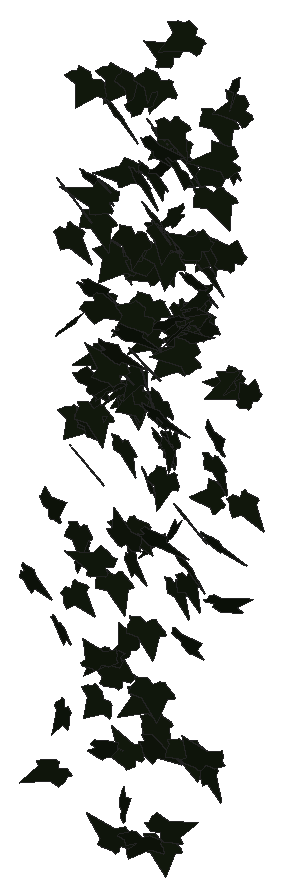
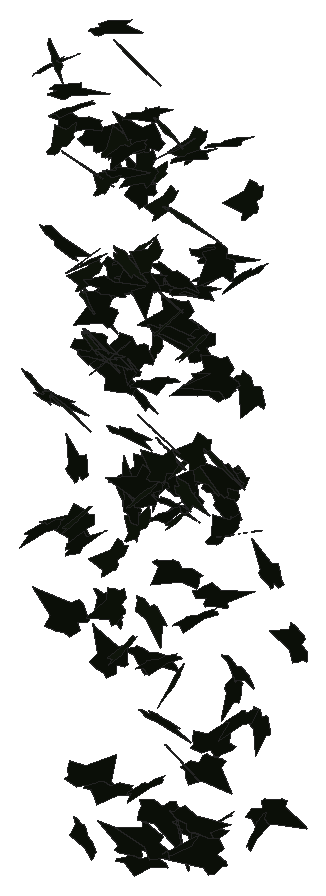
# SketchUp Ruby script. Lengths in inches.
U = 1.inch
M = Sketchup.active_model
def pt(a) = Geom::Point3d.new(a.map { |v| v * U })
def face(e, loops, mat)
  f = e.add_face(loops[0].map { |a| pt(a) })
  loops[1..].each { |l| e.add_face(l.map { |a| pt(a) }).erase! }
  f.material = f.back_material = mat if mat
  f
end
# faces: each face lists its corners as indices into pts; further lists are holes
def faces(e, pts, list, mat = nil) = list.each { |f| face(e, (f[0].is_a?(Array) ? f : [f]).map { |l| l.map { |i| pts[i] } }, mat) }
# xy, xz, yz: faces in a plane at the given z, y or x. An outline is a flat list of corners, or four numbers for a rectangle; further outlines are holes
def ring(l) = l.size == 4 ? [[l[0], l[1]], [l[2], l[1]], [l[2], l[3]], [l[0], l[3]]] : l.each_slice(2).to_a
def flat(e, list, mat, &to3) = list.each { |f| face(e, (f[0].is_a?(Array) ? f : [f]).map { |l| ring(l).map { |u, v| to3.(u, v) } }, mat) }
def xy(e, z, list, mat = nil) = flat(e, list, mat) { |x, y| [x, y, z] }
def xz(e, y, list, mat = nil) = flat(e, list, mat) { |x, z| [x, y, z] }
def yz(e, x, list, mat = nil) = flat(e, list, mat) { |y, z| [x, y, z] }
def lines(e, pts, list) = list.each { |a, b| e.add_line(pt(pts[a]), pt(pts[b])) }
# prism: a flat outline (further loops are holes) pulled along v
def prism(e, loops, v, mat = nil)
  f = face(e, loops, mat); d = Geom::Vector3d.new(v.map { |x| x * U })
  f.pushpull(f.normal.samedirection?(d) ? d.length : -d.length)
end
def box(e, o, s, mat = nil) = prism(e, [[o, [o[0] + s[0], o[1], o[2]], [o[0] + s[0], o[1] + s[1], o[2]], [o[0], o[1] + s[1], o[2]]]], [0, 0, s[2]], mat)
def at(x, y, z, deg = 0) = Geom::Transformation.translation(pt([x, y, z])) * Geom::Transformation.rotation(ORIGIN, Z_AXIS, deg.degrees)
def axes(o, x, y, z) = Geom::Transformation.new([*x, 0, *y, 0, *z, 0, *pt(o).to_a, 1])
def part(name) = M.definitions.add(name)
# library, detail: a bought-in or finely detailed component or shape, given as its bounding box
def library(name, o, s) = part(name).tap { |d| box(d.entities, o, s) }
def detail(e, o, s) = box(e.add_group.entities, o, s)
def put(e, d, t, mat = nil) = e.add_instance(d, t).tap { |i| i.material = mat if mat }
def group(e, t, mat = nil) = e.add_group.tap { |g| g.transformation = t; g.material = mat if mat }.entities
root = M.entities
M.materials.add("1026 AP 7946 SUNNY SIDE UP").color = [254, 231, 186]
M.materials.add("efeu1").color = [18, 25, 13]
c1 = part("ivyleaf_9")
p = [[1.54,2.16,1.25],[1.36,2.04,1.19],[-0.21,0.99,0.68],[-0.71,1.11,0.82],[-0.85,0.86,0.67],[-0.8,0.17,0.21],
  [-0.9,-0.01,0.1],[-0.67,-0.16,-0.02],[-0.08,-0.08,-0.05],[-0.03,-0.6,-0.4],[0.65,-0.88,-0.66],[0.83,-0.6,-0.49],
  [1.29,-0.42,-0.43],[1.8125,-0.07,-0.26],[1.21,0.44,0.15]]
faces(c1.entities,p,[[0,1,2,3,4,5,6,7,8,9,10,11,12,13,14]],"efeu1")
put(root,c1,axes([168.82,210.77,309.2],[-0.44916,-0.2938,0.16947],[0.00239,-0.21881,-0.39713],[0.53074,-0.24766,0.14521]),"1026 AP 7946 SUNNY SIDE UP")
put(root,c1,axes([168.69,210.7,304.06],[-0.41014,-0.05137,-0.32784],[0.50445,-0.00547,-0.27027],[0.04453,-0.41121,0.04211]),"1026 AP 7946 SUNNY SIDE UP")
put(root,c1,axes([168.9375,210.49,303.13],[0.06762,-0.09449,-0.44363],[-0.43394,0.33096,-0.10139],[0.53956,0.27802,-0.02595]),"1026 AP 7946 SUNNY SIDE UP")
put(root,c1,axes([168.94,211.13,324.72],[-0.38736,-0.37553,0.13039],[-0.00621,-0.14914,-0.45698],[0.62417,-0.23454,0.07638]),"1026 AP 7946 SUNNY SIDE UP")
put(root,c1,axes([169.12,209.28,314.23],[0.11699,0.37991,0.23372],[0.10984,0.21488,-0.39682],[-0.6853,0.0993,-0.0237]),"1026 AP 7946 SUNNY SIDE UP")
put(root,c1,axes([169.49,211.05,312.21],[-0.50728,0.27598,0.01138],[-0.05199,-0.02414,-0.43558],[-0.43108,-0.32185,0.03915]),"1026 AP 7946 SUNNY SIDE UP")
put(root,c1,axes([168.85,211.18,320.21],[0.70778,-0.08409,-0.10764],[-0.17067,-0.0163,-0.47045],[0.12289,0.4617,-0.03342]),"1026 AP 7946 SUNNY SIDE UP")
put(root,c1,axes([168.6,207.34,303.48],[0.19237,-0.05459,-0.43971],[0.67578,0.02942,0.12329],[0.02118,-0.44273,0.05977]),"1026 AP 7946 SUNNY SIDE UP")
put(root,c1,axes([168.95,209.93,301.71],[0.16673,-0.27771,-0.32909],[-0.12089,0.30956,-0.30322],[0.6526,0.12829,0.02791]),"1026 AP 7946 SUNNY SIDE UP")
put(root,c1,axes([169.16,210.78,309.1],[-0.26105,-0.17459,0.42549],[0.43389,0.30871,0.24991],[-0.55757,0.32197,-0.00473]),"1026 AP 7946 SUNNY SIDE UP")
put(root,c1,axes([169.3,208.57,300.82],[0.46262,-0.09432,-0.3028],[-0.46182,0.03704,-0.31547],[0.14676,0.41384,-0.03821]),"1026 AP 7946 SUNNY SIDE UP")
put(root,c1,axes([169.2,209.03,296.68],[0.06619,-0.08624,-0.47588],[0.47183,-0.35134,0.09379],[-0.56764,-0.30209,0.02247]),"1026 AP 7946 SUNNY SIDE UP")
put(root,c1,axes([169.07,208.25,306.24],[-0.08274,0.09051,0.45294],[0.28188,-0.40104,0.10494],[0.64624,0.18652,0.01222]),"1026 AP 7946 SUNNY SIDE UP")
put(root,c1,axes([170.04,210.75,319.65],[-0.35867,0.07659,0.42283],[-0.65429,-0.07395,-0.22469],[0.04514,-0.46332,0.1029]),"1026 AP 7946 SUNNY SIDE UP")
put(root,c1,axes([169.01,210.82,315.39],[0.7164,-0.02846,0.14708],[0.2178,-0.06134,-0.46778],[0.07126,0.47354,-0.04893]),"1026 AP 7946 SUNNY SIDE UP")
put(root,c1,axes([169.54,212.35,324.51],[-0.37716,-0.36879,0.16763],[-0.0715,-0.16581,-0.45137],[0.63112,-0.23917,0.04904]),"1026 AP 7946 SUNNY SIDE UP")
put(root,c1,axes([169.26,209.19,318.7],[0.23083,-0.37629,-0.25558],[-0.04868,0.24966,-0.41107],[0.70518,0.14041,0.05528]),"1026 AP 7946 SUNNY SIDE UP")
put(root,c1,axes([169.2,210.66,310.93],[0.04248,0.01106,0.47888],[0.64554,-0.21906,-0.02049],[0.34307,0.41082,-0.02074]),"1026 AP 7946 SUNNY SIDE UP")
put(root,c1,axes([169.54,211.86,316.82],[0.27851,-0.42128,-0.03951],[-0.03604,0.02937,-0.47052],[0.66386,0.17833,-0.00897]),"1026 AP 7946 SUNNY SIDE UP")
put(root,c1,axes([170.4,211.17,297.5],[-0.07447,0.0937,0.44462],[-0.63166,0.16994,-0.08253],[-0.28655,-0.39896,0.06638]),"1026 AP 7946 SUNNY SIDE UP")
put(root,c1,axes([169.56,210,309.45],[-0.11395,0.13878,0.43524],[0.32797,-0.36654,0.15905],[0.61623,0.22074,-0.00417]),"1026 AP 7946 SUNNY SIDE UP")
put(root,c1,axes([169.57,210.67,314.86],[0.15343,-0.11273,-0.46067],[0.19734,0.44567,-0.08505],[0.69674,-0.1014,0.12554]),"1026 AP 7946 SUNNY SIDE UP")
put(root,c1,axes([169.78,210.49,319],[-0.04222,-0.43627,-0.12199],[0.06935,0.11305,-0.44812],[0.70641,-0.03718,0.0367]),"1026 AP 7946 SUNNY SIDE UP")
put(root,c1,axes([170.27,210.48,311.15],[-0.44003,0.25477,-0.30147],[-0.29341,0.23,0.38954],[0.53687,0.33452,-0.0342]),"1026 AP 7946 SUNNY SIDE UP")
put(root,c1,axes([169.58,208.62,321.07],[0.48665,-0.32928,0.15629],[0.11925,-0.13875,-0.46473],[0.55872,0.31642,-0.03693]),"1026 AP 7946 SUNNY SIDE UP")
put(root,c1,axes([170.33,211.67,310.89],[-0.46674,0.20082,-0.2239],[0.18852,-0.20151,-0.35981],[-0.42683,-0.3086,0.08591]),"1026 AP 7946 SUNNY SIDE UP")
put(root,c1,axes([170.25,210.17,296.98],[-0.26999,-0.30602,0.31758],[-0.12609,-0.30532,-0.35804],[0.67325,-0.17991,0.0603]),"1026 AP 7946 SUNNY SIDE UP")
put(root,c1,axes([169.81,211.19,312.21],[0.44671,-0.28655,0.17932],[0.168,-0.14112,-0.41593],[0.5011,0.30276,-0.02041]),"1026 AP 7946 SUNNY SIDE UP")
put(root,c1,axes([170.03,212.05,310.04],[0.18698,-0.40028,0.02422],[-0.00157,-0.02719,-0.43024],[0.6307,0.1186,-0.00825]),"1026 AP 7946 SUNNY SIDE UP")
put(root,c1,axes([170.1875,212.4,324.49],[-0.14005,-0.43833,0.15107],[0.02037,-0.15416,-0.45974],[0.72775,-0.08004,0.04194]),"1026 AP 7946 SUNNY SIDE UP")
put(root,c1,axes([170.65,212.16,310.51],[-0.65902,-0.02284,0.00764],[-0.00631,-0.06356,-0.42785],[0.03729,-0.41434,0.06273]),"1026 AP 7946 SUNNY SIDE UP")
put(root,c1,axes([170.68,210.13,299.26],[0.02566,0.19641,-0.41236],[-0.03444,-0.40083,-0.20531],[-0.70181,0.02685,-0.005]),"1026 AP 7946 SUNNY SIDE UP")
put(root,c1,axes([170.26,209.68,310.57],[-0.0661,-0.46648,-0.09457],[0.03117,0.0877,-0.48185],[0.74612,-0.04499,0.01175]),"1026 AP 7946 SUNNY SIDE UP")
put(root,c1,axes([170.375,212.28,310.21],[-0.10789,-0.42811,-0.02622],[0.01482,0.02181,-0.4465],[0.67397,-0.06901,0.00562]),"1026 AP 7946 SUNNY SIDE UP")
put(root,c1,axes([171.1,211.04,321.17],[-0.52802,0.28324,0.12182],[-0.28695,-0.04598,-0.4265],[-0.38685,-0.3525,0.15009]),"1026 AP 7946 SUNNY SIDE UP")
put(root,c1,axes([170.68,211.92,310.01],[-0.29502,-0.16758,0.36226],[-0.184,-0.34907,-0.23711],[0.58563,-0.1941,0.108]),"1026 AP 7946 SUNNY SIDE UP")
put(root,c1,axes([170.24,210.91,324],[0.4667,-0.36382,0.09632],[0.06315,-0.09038,-0.48352],[0.5881,0.29842,-0.02452]),"1026 AP 7946 SUNNY SIDE UP")
put(root,c1,axes([170.97,206.33,295.73],[-0.065,0.02955,-0.46399],[-0.09455,-0.44877,-0.02726],[-0.70365,0.05757,0.04652]),"1026 AP 7946 SUNNY SIDE UP")
put(root,c1,axes([170.48,212.09,317.57],[0.21293,-0.42426,-0.04286],[-0.05569,0.02977,-0.45792],[0.66763,0.1378,-0.02453]),"1026 AP 7946 SUNNY SIDE UP")
put(root,c1,axes([171.02,209.16,299.35],[0.27068,0.14292,0.38581],[-0.58047,-0.1001,0.21405],[0.24254,-0.39907,0.0817]),"1026 AP 7946 SUNNY SIDE UP")
put(root,c1,axes([170.74,211.35,303.24],[0.40077,-0.2858,-0.27458],[-0.31402,0.17601,-0.39255],[0.52617,0.32274,-0.02513]),"1026 AP 7946 SUNNY SIDE UP")
put(root,c1,axes([171.34,210.62,299.51],[-0.5354,0.10283,-0.27293],[-0.37605,0.12134,0.36507],[0.24297,0.41439,-0.03639]),"1026 AP 7946 SUNNY SIDE UP")
put(root,c1,axes([170.51,212.35,311.78],[0.1541,-0.2759,0.33116],[0.30239,-0.26677,-0.2964],[0.5956,0.20683,0.06481]),"1026 AP 7946 SUNNY SIDE UP")
put(root,c1,axes([171.23,210.25,317.76],[-0.52932,-0.32246,0.09847],[-0.06335,-0.0982,-0.47884],[0.52587,-0.33641,0.04144]),"1026 AP 7946 SUNNY SIDE UP")
put(root,c1,axes([170.67,208.21,309.21],[0.33713,-0.3167,0.25374],[0.21895,-0.20535,-0.3952],[0.59349,0.25566,0.00166]),"1026 AP 7946 SUNNY SIDE UP")
put(root,c1,axes([171.48,212.15,313.26],[-0.62429,0.15843,-0.05617],[0.05584,-0.05981,-0.43859],[-0.25795,-0.39639,0.04098]),"1026 AP 7946 SUNNY SIDE UP")
put(root,c1,axes([171.3,211.28,311.95],[-0.55599,0.02451,-0.23914],[0.34764,-0.10074,-0.35827],[-0.1184,-0.41089,0.07102]),"1026 AP 7946 SUNNY SIDE UP")
put(root,c1,axes([170.77,209.27,295.29],[0.50947,0.11477,0.29764],[0.45534,0.03779,-0.35059],[-0.17517,0.43203,-0.04568]),"1026 AP 7946 SUNNY SIDE UP")
put(root,c1,axes([171.63,211.13,324.51],[-0.57992,0.18717,-0.25185],[-0.30821,0.15359,0.42482],[0.37508,0.4156,-0.04031]),"1026 AP 7946 SUNNY SIDE UP")
put(root,c1,axes([171.87,208.27,304.53],[-0.15581,0.02322,0.4325],[-0.64922,-0.0862,-0.09602],[0.12389,-0.42253,0.04078]),"1026 AP 7946 SUNNY SIDE UP")
put(root,c1,axes([171.37,212.04,314.89],[-0.31506,-0.39298,-0.03477],[0.05023,0.01906,-0.45387],[0.61787,-0.20194,0.01916]),"1026 AP 7946 SUNNY SIDE UP")
put(root,c1,axes([171.875,209.13,313.08],[-0.48691,-0.33151,-0.03945],[-0.07115,-0.00747,0.46641],[-0.51955,0.3117,-0.0269]),"1026 AP 7946 SUNNY SIDE UP")
put(root,c1,axes([171.46,210.77,318.58],[-0.54471,-0.13535,-0.2828],[0.42534,0.05612,-0.3809],[0.22285,-0.43794,0.03574]),"1026 AP 7946 SUNNY SIDE UP")
put(root,c1,axes([171.77,212.01,325.28],[-0.35852,-0.40447,0.03951],[0.01331,-0.05133,-0.47746],[0.63905,-0.22584,0.03212]),"1026 AP 7946 SUNNY SIDE UP")
put(root,c1,axes([171.64,212.29,310.29],[-0.0655,-0.35554,0.25285],[0.005,-0.24884,-0.36923],[0.68111,-0.03236,0.02703]),"1026 AP 7946 SUNNY SIDE UP")
put(root,c1,axes([171.51,211.88,323.18],[0.62505,-0.2407,-0.0636],[-0.10176,0.00951,-0.47798],[0.37671,0.40196,-0.02358]),"1026 AP 7946 SUNNY SIDE UP")
put(root,c1,axes([172.16,209.81,295.08],[-0.38375,-0.34946,0.12221],[0.08538,0.10907,0.43939],[-0.57499,0.24943,-0.01632]),"1026 AP 7946 SUNNY SIDE UP")
put(root,c1,axes([171.54,210.94,321.29],[0.33508,-0.38797,0.1093],[0.05672,-0.10364,-0.45624],[0.63082,0.2154,-0.01703]),"1026 AP 7946 SUNNY SIDE UP")
put(root,c1,axes([172.13,211.7,318.59],[0.4587,0.07076,-0.35299],[-0.52246,-0.08538,-0.30972],[-0.1743,0.44214,-0.00057]),"1026 AP 7946 SUNNY SIDE UP")
put(root,c1,axes([171.71,211.6,319.29],[0.27146,-0.34768,0.24496],[0.15324,-0.21922,-0.40109],[0.64616,0.19806,-0.00779]),"1026 AP 7946 SUNNY SIDE UP")
put(root,c1,axes([172.75,211.54,326.98],[-0.28748,0.30603,0.33505],[-0.33928,0.24502,-0.36299],[-0.61252,-0.27935,0.04381]),"1026 AP 7946 SUNNY SIDE UP")
put(root,c1,axes([172.51,209.93,315.61],[-0.68647,-0.11417,0.03279],[-0.03283,-0.04798,-0.46323],[0.18373,-0.43514,0.03972]),"1026 AP 7946 SUNNY SIDE UP")
put(root,c1,axes([172.75,210.64,317.66],[-0.51442,0.00429,0.30625],[-0.4647,-0.05254,-0.33462],[0.0506,-0.43889,0.04045]),"1026 AP 7946 SUNNY SIDE UP")
put(root,c1,axes([172.5,212.22,312.64],[-0.63756,-0.12658,-0.00105],[0.0197,-0.03912,-0.43577],[0.19806,-0.40358,0.03996]),"1026 AP 7946 SUNNY SIDE UP")
put(root,c1,axes([172.08,208.65,303.92],[-0.04054,-0.46347,-0.12287],[0.0475,0.11499,-0.47694],[0.74999,-0.03234,0.02356]),"1026 AP 7946 SUNNY SIDE UP")
put(root,c1,axes([172.6,212.23,322.78],[-0.61513,-0.20902,0.12115],[-0.12157,-0.10545,-0.45407],[0.35796,-0.39501,0.05398]),"1026 AP 7946 SUNNY SIDE UP")
put(root,c1,axes([172.64,212.13,319.38],[-0.55172,0.21683,-0.17388],[0.12901,-0.18057,-0.41275],[-0.4136,-0.34557,0.1032]),"1026 AP 7946 SUNNY SIDE UP")
put(root,c1,axes([172.01,211.85,308.8],[0.17934,-0.36307,0.27866],[0.1231,-0.26108,-0.39357],[0.70316,0.13831,-0.00217]),"1026 AP 7946 SUNNY SIDE UP")
put(root,c1,axes([171.83,211.46,310.13],[0.44883,-0.19012,0.32937],[0.41744,-0.1801,-0.35437],[0.41177,0.38981,0.00023]),"1026 AP 7946 SUNNY SIDE UP")
put(root,c1,axes([172.7,210.41,304.78],[-0.11046,0.42947,0.13083],[-0.04035,0.12201,-0.44757],[-0.70197,-0.07459,0.00514]),"1026 AP 7946 SUNNY SIDE UP")
put(root,c1,axes([172.28,211.16,321.58],[0.22798,0.43409,0.15482],[-0.21831,-0.1062,0.46096],[0.68722,-0.17775,0.09507]),"1026 AP 7946 SUNNY SIDE UP")
put(root,c1,axes([172.16,209.43,306.09],[-0.16256,-0.19461,-0.40075],[0.37592,0.30726,-0.22265],[0.56952,-0.25836,0.03258]),"1026 AP 7946 SUNNY SIDE UP")
put(root,c1,axes([172.95,210.43,317.65],[-0.59882,0.22327,0.03665],[-0.08702,-0.02701,-0.45188],[-0.34437,-0.38142,0.05045]),"1026 AP 7946 SUNNY SIDE UP")
put(root,c1,axes([171.93,208.4375,314.47],[0.47038,-0.10942,0.34003],[0.46188,-0.15503,-0.3275],[0.29436,0.4181,-0.0295]),"1026 AP 7946 SUNNY SIDE UP")
put(root,c1,axes([172.25,209.04,309.99],[0.17828,-0.42678,0.07941],[0.02504,-0.07803,-0.45535],[0.68216,0.1144,-0.00404]),"1026 AP 7946 SUNNY SIDE UP")
put(root,c1,axes([172.9,211.18,309.31],[0.3,-0.07088,-0.41405],[-0.62494,0.06658,-0.20628],[0.14305,0.43953,-0.03283]),"1026 AP 7946 SUNNY SIDE UP")
put(root,c1,axes([172.48,211.88,323.61],[0.04856,-0.42018,-0.22143],[-0.04164,0.21112,-0.43268],[0.73924,0.03949,-0.00982]),"1026 AP 7946 SUNNY SIDE UP")
put(root,c1,axes([172.48,211.09,318.1875],[-0.20009,-0.38963,-0.25495],[0.22164,0.20927,-0.41661],[0.68917,-0.18043,0.05996]),"1026 AP 7946 SUNNY SIDE UP")
put(root,c1,axes([172.43,210.7,321.78],[0.04441,-0.3824,0.27245],[0.19782,-0.25096,-0.38598],[0.70583,0.0944,0.09103]),"1026 AP 7946 SUNNY SIDE UP")
put(root,c1,axes([173.42,212.14,317.89],[-0.22794,0.13106,0.43301],[-0.69035,-0.02157,-0.14945],[-0.0338,-0.44339,0.13243]),"1026 AP 7946 SUNNY SIDE UP")
put(root,c1,axes([173.03,210.82,315.12],[0.25155,0.41027,0.01339],[0.04018,0.00147,-0.45301],[-0.64408,0.16033,-0.02303]),"1026 AP 7946 SUNNY SIDE UP")
put(root,c1,axes([172.8,210.95,319.01],[-0.05739,-0.4132,0.21565],[0.0025,-0.21243,-0.42817],[0.73,-0.03176,0.01842]),"1026 AP 7946 SUNNY SIDE UP")
put(root,c1,axes([172.45,210.33,295.67],[0.24588,-0.07082,-0.42348],[0.61385,0.17836,0.1225],[0.22925,-0.40161,0.1262]),"1026 AP 7946 SUNNY SIDE UP")
put(root,c1,axes([172.55,208.65,315.46],[0.64227,0.01302,0.20717],[0.3167,-0.01808,-0.42051],[-0.00579,0.45489,-0.01998]),"1026 AP 7946 SUNNY SIDE UP")
put(root,c1,axes([172.66,212.16,305.69],[0.58621,-0.27248,0.03448],[0.01056,-0.04998,-0.47453],[0.43184,0.3711,-0.0352]),"1026 AP 7946 SUNNY SIDE UP")
put(root,c1,axes([172.99,211.23,309.55],[-0.38901,-0.01093,-0.39282],[0.58515,-0.10643,-0.24626],[-0.13133,-0.44184,0.0663]),"1026 AP 7946 SUNNY SIDE UP")
put(root,c1,axes([172.94,208.13,293.75],[-0.00472,0.17792,0.44699],[0.01524,-0.43278,0.18079],[0.73576,0.01011,-0.00088]),"1026 AP 7946 SUNNY SIDE UP")
put(root,c1,axes([172.68,210.57,323],[0.06132,-0.10165,0.46078],[0.52143,-0.30471,-0.10278],[0.49956,0.33053,0.05072]),"1026 AP 7946 SUNNY SIDE UP")
put(root,c1,axes([173.52,211.96,328],[-0.50009,-0.24362,0.25137],[-0.27457,-0.17461,-0.41276],[0.46929,-0.36177,0.02638]),"1026 AP 7946 SUNNY SIDE UP")
put(root,c1,axes([173.04,211.78,315.34],[0.32847,-0.36432,-0.21333],[-0.10686,0.19654,-0.42999],[0.64858,0.21689,0.0372]),"1026 AP 7946 SUNNY SIDE UP")
put(root,c1,axes([173.07,212.16,322.12],[0.17143,-0.38303,0.23553],[0.13403,-0.21541,-0.41102],[0.69027,0.13695,0.02131]),"1026 AP 7946 SUNNY SIDE UP")
put(root,c1,axes([172.9,211.35,314.21],[0.49904,0.14532,-0.30767],[0.2952,0.26354,0.33825],[0.43221,-0.34779,0.1242]),"1026 AP 7946 SUNNY SIDE UP")
put(root,c1,axes([173.35,210.52,318.45],[-0.22383,-0.45679,0.01025],[0.01474,-0.01605,-0.49279],[0.71838,-0.142,0.01331]),"1026 AP 7946 SUNNY SIDE UP")
put(root,c1,axes([173.35,209.16,301.97],[-0.10403,-0.4478,-0.09322],[0.0492,0.0842,-0.46545],[0.71588,-0.07086,0.01844]),"1026 AP 7946 SUNNY SIDE UP")
put(root,c1,axes([173.74,208.76,309.02],[0.3609,-0.05172,-0.37952],[-0.55204,0.11201,-0.24107],[0.19208,0.41909,0.02026]),"1026 AP 7946 SUNNY SIDE UP")
put(root,c1,axes([173.39,209.6875,297.34],[0.1101,-0.41426,-0.17979],[-0.01358,0.17298,-0.43137],[0.70527,0.068,0.01976]),"1026 AP 7946 SUNNY SIDE UP")
put(root,c1,axes([173.85,212.13,315.2],[-0.59776,-0.21172,0.04382],[-0.01619,-0.07065,-0.4449],[0.33955,-0.37609,0.05594]),"1026 AP 7946 SUNNY SIDE UP")
put(root,c1,axes([173.48,210.85,303.1],[0.24093,-0.41674,0.03042],[-0.01159,-0.03666,-0.45719],[0.65709,0.15216,-0.01922]),"1026 AP 7946 SUNNY SIDE UP")
put(root,c1,axes([174.13,211.73,315.52],[-0.61894,0.18605,-0.05832],[0.04811,-0.06936,-0.44606],[-0.30247,-0.39174,0.0484]),"1026 AP 7946 SUNNY SIDE UP")
put(root,c1,axes([174.32,206.17,293.47],[0.04859,0.03022,0.47605],[-0.61614,0.2482,0.01173],[-0.38755,-0.39081,0.04104]),"1026 AP 7946 SUNNY SIDE UP")
put(root,c1,axes([174.18,208.4,299.17],[-0.72174,0.00966,0.00612],[-0.0107,-0.04514,-0.47093],[-0.0142,-0.45682,0.04397]),"1026 AP 7946 SUNNY SIDE UP")
put(root,c1,axes([174.43,211.73,315.24],[-0.16282,0.06548,-0.44334],[-0.55651,-0.27081,0.04366],[-0.39948,0.35058,0.11988]),"1026 AP 7946 SUNNY SIDE UP")
put(root,c1,axes([173.53,211.72,316.91],[0.67551,-0.10326,0.00913],[-0.00052,-0.04164,-0.4535],[0.16304,0.42768,-0.03928]),"1026 AP 7946 SUNNY SIDE UP")
put(root,c1,axes([174.23,211.88,315.54],[-0.54041,0.26156,-0.0789],[0.06076,-0.07765,-0.44369],[-0.42489,-0.34378,0.03691]),"1026 AP 7946 SUNNY SIDE UP")
put(root,c1,axes([174.2,206.76,307.14],[0.42452,-0.11065,0.36869],[-0.34065,0.31465,0.26995],[-0.48169,-0.32003,0.13403]),"1026 AP 7946 SUNNY SIDE UP")
put(root,c1,axes([173.91,210.69,322.51],[-0.06068,-0.31351,0.36269],[0.15073,-0.35284,-0.31335],[0.72792,0.04693,0.09512]),"1026 AP 7946 SUNNY SIDE UP")
put(root,c1,axes([174.1,208.28,313.56],[0.02361,-0.09543,0.46734],[0.03019,-0.45391,-0.10156],[0.72914,0.02188,-0.01093]),"1026 AP 7946 SUNNY SIDE UP")
put(root,c1,axes([174.71,211.33,316.72],[-0.49389,0.29884,-0.08786],[0.06609,-0.08172,-0.44607],[-0.48491,-0.31551,0.02869]),"1026 AP 7946 SUNNY SIDE UP")
put(root,c1,axes([174.375,212.0625,318.41],[-0.27084,-0.34064,0.23454],[-0.07806,-0.22988,-0.39107],[0.6412,-0.17187,0.05146]),"1026 AP 7946 SUNNY SIDE UP")
put(root,c1,axes([174.25,212.14,318.65],[0.04182,-0.43987,0.06862],[-0.00822,-0.06953,-0.45428],[0.70008,0.02546,-0.00944]),"1026 AP 7946 SUNNY SIDE UP")
put(root,c1,axes([174.89,211.86,322.29],[-0.71497,0.07911,-0.03156],[0.02078,-0.10131,-0.46536],[-0.13202,-0.44436,0.09766]),"1026 AP 7946 SUNNY SIDE UP")
put(root,c1,axes([174.36,212.25,308.54],[0.19869,-0.41942,0.00888],[-0.01833,-0.015,-0.45107],[0.65947,0.12595,-0.01522]),"1026 AP 7946 SUNNY SIDE UP")
put(root,c1,axes([174.85,211.98,307.1],[-0.19412,-0.08487,0.42423],[-0.41814,-0.31732,-0.15118],[0.51304,-0.29073,0.0373]),"1026 AP 7946 SUNNY SIDE UP")
put(root,c1,axes([174.27,211.6875,317.84],[0.31263,-0.37555,0.13069],[0.10752,-0.10972,-0.43831],[0.61505,0.21008,0.01019]),"1026 AP 7946 SUNNY SIDE UP")
put(root,c1,axes([174.65,212.21,324.5625],[-0.05263,-0.46918,-0.07239],[0.10901,0.06219,-0.4797],[0.73735,-0.04268,0.06575]),"1026 AP 7946 SUNNY SIDE UP")
put(root,c1,axes([174.68,210.13,304.12],[-0.23155,-0.04246,-0.42204],[0.64374,0.03007,-0.15473],[0.06725,-0.43407,0.02799]),"1026 AP 7946 SUNNY SIDE UP")
put(root,c1,axes([175.56,211.97,312.74],[-0.45,0.29796,0.1159],[-0.17675,0.04461,-0.42241],[-0.46756,-0.30363,0.04814]),"1026 AP 7946 SUNNY SIDE UP")
put(root,c1,axes([174.83,211.69,309.91],[-0.07615,-0.00908,0.46572],[0.20153,-0.43634,0.00256],[0.6819,0.12794,0.05125]),"1026 AP 7946 SUNNY SIDE UP")
put(root,c1,axes([175.01,209.7,296.6875],[-0.22686,-0.35621,-0.24378],[0.18917,0.20363,-0.39353],[0.64345,-0.18546,0.02975]),"1026 AP 7946 SUNNY SIDE UP")
put(root,c1,axes([175.07,207.98,293.05],[-0.30801,-0.34818,-0.18637],[0.18667,0.13783,-0.40937],[0.58656,-0.2267,0.03241]),"1026 AP 7946 SUNNY SIDE UP")
put(root,c1,axes([175.47,206.22,294.13],[0.364,0.24028,-0.33936],[-0.31423,-0.26511,-0.34402],[-0.56082,0.30449,-0.0275]),"1026 AP 7946 SUNNY SIDE UP")
put(root,c1,axes([175.55,208.71,316.61],[-0.28472,0.36352,-0.2258],[0.12968,-0.2059,-0.41927],[-0.65645,-0.19834,0.01511]),"1026 AP 7946 SUNNY SIDE UP")
put(root,c1,axes([174.88,209.6,301.52],[0.64123,-0.10551,-0.19582],[0.31592,0.03182,0.42739],[-0.12842,-0.44855,0.0736]),"1026 AP 7946 SUNNY SIDE UP")
put(root,c1,axes([175.89,211.56,318.59],[-0.13996,0.18054,0.43815],[-0.48035,0.30058,-0.19603],[-0.54308,-0.31239,0.06047]),"1026 AP 7946 SUNNY SIDE UP")
put(root,c1,axes([175.29,207.18,300.67],[-0.45894,-0.2442,-0.28023],[0.35599,0.15028,-0.39035],[0.44922,-0.36858,0.02305]),"1026 AP 7946 SUNNY SIDE UP")
put(root,c1,axes([175,209.4,305.45],[0.3863,-0.37886,0.15665],[0.11888,-0.13473,-0.46586],[0.63209,0.25687,-0.00812]),"1026 AP 7946 SUNNY SIDE UP")
put(root,c1,axes([175.07,208.02,293.47],[-0.09231,0.06712,0.44206],[0.66349,-0.09217,0.07385],[0.15929,0.4228,-0.05143]),"1026 AP 7946 SUNNY SIDE UP")
put(root,c1,axes([175.95,208.85,315.38],[-0.44997,-0.06691,0.3646],[-0.46505,-0.21514,-0.28922],[0.32426,-0.40141,0.09115]),"1026 AP 7946 SUNNY SIDE UP")
put(root,c1,axes([175.15,210.86,295.19],[-0.11161,-0.07721,-0.45924],[0.70977,-0.03518,-0.06804],[-0.03637,-0.44959,0.08146]),"1026 AP 7946 SUNNY SIDE UP")
put(root,c1,axes([175.44,208.08,307.21],[0.16058,0.28518,0.33162],[-0.21167,-0.29128,0.3097],[0.64023,-0.16783,0.01922]),"1026 AP 7946 SUNNY SIDE UP")
put(root,c1,axes([175.93,211.98,312.69],[-0.65679,-0.05567,0.10537],[-0.14797,-0.06498,-0.43136],[0.10861,-0.42517,0.04954]),"1026 AP 7946 SUNNY SIDE UP")
put(root,c1,axes([175.3,212.01,322.79],[0.02602,-0.32599,0.34273],[0.11014,-0.32923,-0.336],[0.72617,0.06161,0.03868]),"1026 AP 7946 SUNNY SIDE UP")
put(root,c1,axes([175.47,212.28,326.3125],[-0.31857,-0.00058,-0.4449],[0.59046,-0.23581,-0.18254],[-0.33535,-0.41465,0.10123]),"1026 AP 7946 SUNNY SIDE UP")
put(root,c1,axes([175.11,207.04,307.63],[0.65309,-0.03039,0.21707],[0.32178,-0.07167,-0.42629],[0.09322,0.46026,-0.04928]),"1026 AP 7946 SUNNY SIDE UP")
put(root,c1,axes([176.09,209.53,296.35],[0.35973,0.04557,0.41751],[-0.64055,0.01108,0.23584],[0.01999,-0.46503,0.04379]),"1026 AP 7946 SUNNY SIDE UP")
put(root,c1,axes([176.1,212.02,325.47],[-0.37751,-0.12647,0.3939],[-0.30567,-0.35433,-0.2481],[0.55581,-0.28077,0.13109]),"1026 AP 7946 SUNNY SIDE UP")
put(root,c1,axes([176.51,210.64,323.86],[-0.49267,-0.08384,0.3497],[-0.46112,-0.18635,-0.32691],[0.30074,-0.42308,0.07164]),"1026 AP 7946 SUNNY SIDE UP")
put(root,c1,axes([176.1,207.04,310.71],[-0.57573,-0.03944,-0.30063],[0.46265,-0.05459,-0.37332],[-0.00549,-0.46488,0.06657]),"1026 AP 7946 SUNNY SIDE UP")
put(root,c1,axes([176.07,211.89,307.52],[0.16119,-0.36352,-0.27347],[-0.03971,0.26507,-0.38547],[0.70475,0.09808,0.04083]),"1026 AP 7946 SUNNY SIDE UP")
put(root,c1,axes([176.6875,208.42,320.78],[0.03304,0.04879,0.48482],[-0.65117,-0.22534,0.04182],[0.35887,-0.41337,0.03125]),"1026 AP 7946 SUNNY SIDE UP")
put(root,c1,axes([175.92,210.51,303.23],[0.57164,0.23146,-0.1506],[0.16286,0.11101,0.44309],[0.39966,-0.3763,0.03485]),"1026 AP 7946 SUNNY SIDE UP")
put(root,c1,axes([176.87,211.51,312.58],[-0.15741,0.21534,0.37305],[-0.3117,0.30294,-0.24109],[-0.58269,-0.22022,0.02819]),"1026 AP 7946 SUNNY SIDE UP")
put(root,c1,axes([176.24,209.91,322.55],[-0.22267,-0.3381,-0.29716],[0.30111,0.22459,-0.3692],[0.62845,-0.2274,0.07161]),"1026 AP 7946 SUNNY SIDE UP")
put(root,c1,axes([176.07,209.84,306.5],[0.51107,-0.20355,0.24905],[0.34112,-0.11074,-0.39529],[0.36327,0.39036,0.02081]),"1026 AP 7946 SUNNY SIDE UP")
